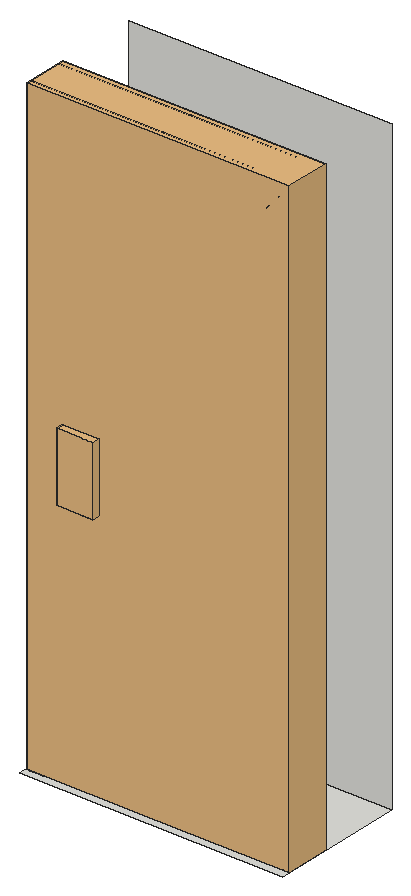
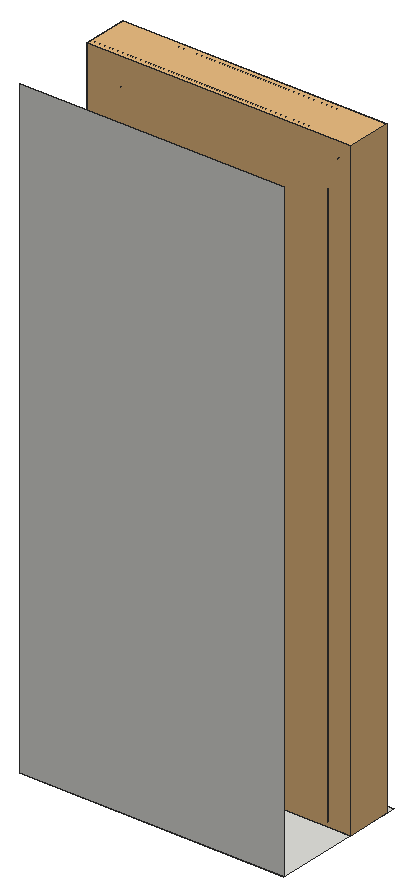
# SketchUp Ruby script. Lengths in inches.
U = 1.inch
M = Sketchup.active_model
def pt(a) = Geom::Point3d.new(a.map { |v| v * U })
def face(e, loops, mat)
  f = e.add_face(loops[0].map { |a| pt(a) })
  loops[1..].each { |l| e.add_face(l.map { |a| pt(a) }).erase! }
  f.material = f.back_material = mat if mat
  f
end
# faces: each face lists its corners as indices into pts; further lists are holes
def faces(e, pts, list, mat = nil) = list.each { |f| face(e, (f[0].is_a?(Array) ? f : [f]).map { |l| l.map { |i| pts[i] } }, mat) }
# xy, xz, yz: faces in a plane at the given z, y or x. An outline is a flat list of corners, or four numbers for a rectangle; further outlines are holes
def ring(l) = l.size == 4 ? [[l[0], l[1]], [l[2], l[1]], [l[2], l[3]], [l[0], l[3]]] : l.each_slice(2).to_a
def flat(e, list, mat, &to3) = list.each { |f| face(e, (f[0].is_a?(Array) ? f : [f]).map { |l| ring(l).map { |u, v| to3.(u, v) } }, mat) }
def xy(e, z, list, mat = nil) = flat(e, list, mat) { |x, y| [x, y, z] }
def xz(e, y, list, mat = nil) = flat(e, list, mat) { |x, z| [x, y, z] }
def yz(e, x, list, mat = nil) = flat(e, list, mat) { |y, z| [x, y, z] }
def lines(e, pts, list) = list.each { |a, b| e.add_line(pt(pts[a]), pt(pts[b])) }
# prism: a flat outline (further loops are holes) pulled along v
def prism(e, loops, v, mat = nil)
  f = face(e, loops, mat); d = Geom::Vector3d.new(v.map { |x| x * U })
  f.pushpull(f.normal.samedirection?(d) ? d.length : -d.length)
end
def box(e, o, s, mat = nil) = prism(e, [[o, [o[0] + s[0], o[1], o[2]], [o[0] + s[0], o[1] + s[1], o[2]], [o[0], o[1] + s[1], o[2]]]], [0, 0, s[2]], mat)
def at(x, y, z, deg = 0) = Geom::Transformation.translation(pt([x, y, z])) * Geom::Transformation.rotation(ORIGIN, Z_AXIS, deg.degrees)
def axes(o, x, y, z) = Geom::Transformation.new([*x, 0, *y, 0, *z, 0, *pt(o).to_a, 1])
def part(name) = M.definitions.add(name)
# library, detail: a bought-in or finely detailed component or shape, given as its bounding box
def library(name, o, s) = part(name).tap { |d| box(d.entities, o, s) }
def detail(e, o, s) = box(e.add_group.entities, o, s)
def put(e, d, t, mat = nil) = e.add_instance(d, t).tap { |i| i.material = mat if mat }
def group(e, t, mat = nil) = e.add_group.tap { |g| g.transformation = t; g.material = mat if mat }.entities
root = M.entities
M.materials.add("Material \#0").color = [86, 53, 35]
M.materials.add("Material \#1").color = [140, 140, 140]
c1 = library("3DGeom~3_Defintion",[-83.33,-500,-350],[620.1,1000,533.33])
c2 = part("3DGeom~18_Defintion")
xz(c2.entities,-241.71,[[-976.3,0,23.7,0,23.7,7.58],[-976.3,0,23.7,7.58,-976.3,7.58]],"Material \#0")
xz(c2.entities,241.71,[[-976.3,0,-976.3,7.58,23.7,7.58],[-976.3,0,23.7,7.58,23.7,0]],"Material \#0")
yz(c2.entities,23.7,[[-241.71,0,0,0,-241.71,7.58],[0,0,0,7.58,-241.71,7.58],[0,0,241.71,0,241.71,7.58],[0,0,241.71,7.58,0,7.58]],"Material \#0")
c3 = part("3DGeom~20_Defintion")
xy(c3.entities,0,[[-976.3,-241.71,-976.3,-223.46,23.7,-241.71],[23.7,-241.71,-976.3,-223.46,5.45,-223.46],[23.7,-241.71,5.45,-223.46,5.45,0],[23.7,-241.71,5.45,0,23.7,0],[-976.3,-223.46,-976.3,-211.85,5.45,-223.46],
  [5.45,-223.46,-976.3,-211.85,-6.16,-211.85],[5.45,-223.46,-6.16,-211.85,-6.16,0],[5.45,-223.46,-6.16,0,5.45,0],[-6.16,0,-6.16,211.85,5.45,223.46],[-6.16,0,5.45,223.46,5.45,0],
  [5.45,0,23.7,241.71,23.7,0],[5.45,0,5.45,223.46,23.7,241.71],[-976.3,211.85,-976.3,223.46,5.45,223.46],[-976.3,211.85,5.45,223.46,-6.16,211.85],[-976.3,223.46,-976.3,241.71,23.7,241.71],
  [-976.3,223.46,23.7,241.71,5.45,223.46]],"Material \#0")
c4 = part("3DGeom~22_Defintion")
xz(c4.entities,-210.625,[[-1016.13,2.47,-1016.13,9.96,-16.28,2.47],[-16.28,2.47,-1016.13,9.96,-16.28,9.96],[-1016.13,9.96,-1016.13,51.7,-16.28,51.7],[-1016.13,9.96,-16.28,51.7,-16.28,9.96],[-1016.13,51.7,-1016.13,72.71,-16.28,51.7]],"Material \#0")
xz(c4.entities,210.625,[[-1016.13,2.47,-16.28,2.47,-1016.13,9.96],[-16.28,2.47,-16.28,9.96,-1016.13,9.96],[-1016.13,9.96,-16.28,51.7,-1016.13,51.7],[-1016.13,9.96,-16.28,9.96,-16.28,51.7],[-1016.13,51.7,-16.28,51.7,-1016.13,72.71]],"Material \#0")
yz(c4.entities,-16.28,[[-210.625,2.47,-210.625,9.96,0,9.96],[-210.625,2.47,0,9.96,0,2.47],[0,2.47,0,9.96,210.625,2.47],[210.625,2.47,0,9.96,210.625,9.96],[-210.625,9.96,-210.625,51.7,0,51.7],
  [-210.625,9.96,0,51.7,0,9.96],[0,9.96,0,51.7,210.625,9.96],[210.625,9.96,0,51.7,210.625,51.7],[-210.625,51.7,0,72.71,0,51.7],[0,51.7,0,72.71,210.625,51.7]],"Material \#0")
p = [[-1016.13,-210.625,72.71],[-16.13,-210.77,73.09],[-16.28,-210.625,51.7],[-16.28,-210.625,51.7],[-16.13,-210.77,73.09],[-16.28,0,72.71],
  [-16.13,210.77,73.09],[-16.28,210.625,51.7],[-16.28,210.625,51.7],[-16.13,210.77,73.09],[-1016.13,210.625,72.71]]
faces(c4.entities,p,[[0,1,2],[3,4,5],[5,6,7],[8,9,10]],"Material \#0")
c5 = part("3DGeom~21_Defintion")
xy(c5.entities,73.08,[[-976.3,-241.71,23.7,-241.71,-976.3,-223.46],[23.7,-241.71,5.45,-223.46,-976.3,-223.46],[23.7,-241.71,23.7,0,5.45,-223.46],[5.45,-223.46,23.7,0,5.45,0],[23.7,0,23.7,241.71,5.45,223.46],
  [5.45,0,23.7,0,5.45,223.46],[-976.3,223.46,23.7,241.71,-976.3,241.71],[-976.3,223.46,5.45,223.46,23.7,241.71]],"Material \#0")
c6 = part("3DGeom~19_Defintion")
xy(c6.entities,0,[[-6.28,-215.79,-994.45,-208.55,-13.52,-208.55],[-994.45,-215.79,-994.45,-208.55,-6.28,-215.79],[-6.28,-215.79,-13.52,-208.55,-13.52,0],[-6.28,-215.79,-13.52,0,-6.28,0],[-13.52,0,-13.52,208.55,-6.28,215.79],
  [-13.52,0,-6.28,215.79,-6.28,0],[-994.45,208.55,-6.28,215.79,-13.52,208.55],[-994.45,208.55,-994.45,215.79,-6.28,215.79]],"Material \#0")
p = [[-13.52,-208.55,0],[-994.45,-208.55,0],[-994.45,-207.81,0.07],[-14.25,-207.81,0.07],[-13.52,-208.55,0],[-14.25,-207.81,0.07],
  [-14.25,0,0.07],[-13.52,0,0],[-13.52,208.55,0],[-14.25,207.81,0.07],[-13.52,208.55,0],[-14.25,207.81,0.07],
  [-994.45,207.81,0.07],[-994.45,208.55,0],[-994.45,-207.21,0.27],[-994.45,-207.21,0.27],[-14.86,-207.21,0.27],[-14.86,-207.21,0.27],
  [-14.86,0,0.27],[-14.86,0,0.27],[-14.86,0,0.27],[-14.86,0,0.27],[-14.86,207.21,0.27],[-14.86,207.21,0.27],
  [-994.45,207.21,0.27],[-994.45,207.21,0.27],[-14.86,-207.21,0.27],[-994.45,-207.21,0.27],[-994.45,-206.74,0.6],[-15.33,-206.74,0.6],
  [-14.86,-207.21,0.27],[-15.33,-206.74,0.6],[-15.33,0,0.6],[-14.86,0,0.27],[-14.86,207.21,0.27],[-15.33,206.74,0.6],
  [-14.86,207.21,0.27],[-15.33,206.74,0.6],[-994.45,206.74,0.6],[-994.45,207.21,0.27],[-994.45,-206.4,1.07],[-15.66,-206.4,1.07],
  [-15.66,-206.4,1.07],[-15.66,0,1.07],[-15.66,206.4,1.07],[-15.66,206.4,1.07],[-994.45,206.4,1.07],[-994.45,-206.2,1.68],
  [-15.86,-206.2,1.68],[-15.86,-206.2,1.68],[-15.86,0,1.68],[-15.86,206.2,1.68],[-15.86,206.2,1.68],[-994.45,206.2,1.68],
  [-994.45,-206.13,2.41],[-15.93,-206.13,2.41],[-15.93,-206.13,2.41],[-15.93,0,2.41],[-15.93,206.13,2.41],[-15.93,206.13,2.41],
  [-994.45,206.13,2.41],[-994.45,-206.13,71.16],[-994.45,-206.22,71.59],[-15.79,-206.28,71.53],[-15.79,-206.28,71.53],[-15.84,0,71.59],
  [-15.93,0,71.16],[-15.79,206.28,71.53],[-15.79,206.28,71.53],[-994.45,206.22,71.59],[-994.45,206.13,71.16],[-15.79,-206.28,71.53],
  [-994.45,-206.48,71.84],[-994.45,-206.9,71.93],[-15.16,-206.9,71.93],[-15.79,-206.28,71.53],[-15.79,-206.28,71.53],[-15.16,-206.9,71.93],
  [-15.16,0,71.93],[-994.45,-206.48,71.84],[-15.59,0,71.84],[-15.79,-206.28,71.53],[-15.59,0,71.84],[-15.79,206.28,71.53],
  [-15.16,206.9,71.93],[-15.59,0,71.84],[-15.79,206.28,71.53],[-994.45,206.48,71.84],[-15.79,206.28,71.53],[-15.16,206.9,71.93],
  [-994.45,206.9,71.93],[-994.45,206.48,71.84],[-15.79,206.28,71.53],[-994.45,-227.27,72.01],[5.41,-227.47,72.33],[4.78,-226.84,71.93],
  [4.78,-226.84,71.93],[5.41,-227.47,72.33],[5.21,0,72.01],[-994.45,-226.84,71.93],[-994.45,-227.27,72.01],[5.21,0,72.01],
  [4.78,0,71.93],[4.78,226.84,71.93],[5.21,0,72.01],[5.21,0,72.01],[5.41,227.47,72.33],[4.78,226.84,71.93],
  [5.41,227.47,72.33],[-994.45,227.27,72.01],[-994.45,227.27,72.01],[-994.45,226.84,71.93],[-994.45,-227.27,72.01],[-994.45,-227.53,72.27],
  [5.41,-227.47,72.33],[5.41,-227.47,72.33],[5.47,0,72.27],[5.21,0,72.01],[5.41,227.47,72.33],[5.41,227.47,72.33],
  [-994.45,227.53,72.27],[-994.45,227.27,72.01],[-994.45,-227.61,72.7],[-994.45,-227.61,74.4375],[-994.45,-227.61,74.4375],[5.55,-227.61,74.4375],
  [5.55,-227.61,74.4375],[5.55,0,74.4375],[5.55,0,72.7],[5.55,227.61,74.4375],[5.55,227.61,74.4375],[-994.45,227.61,74.4375],
  [-994.45,227.61,74.4375],[-994.45,227.61,72.7]]
faces(c6.entities,p,[[0,1,2],[2,3,0],[4,5,6],[6,7,4],[8,7,6],[6,9,8],[10,11,12],[12,13,10],
  [3,2,14],[15,16,3],[5,17,18],[19,6,5],[9,6,20],[21,22,9],[11,23,24],[25,12,11],
  [26,27,28],[28,29,26],[30,31,32],[32,33,30],[34,33,32],[32,35,34],[36,37,38],[38,39,36],
  [29,28,40],[40,41,29],[31,42,43],[43,32,31],[35,32,43],[43,44,35],[37,45,46],[46,38,37],
  [41,40,47],[47,48,41],[42,49,50],[50,43,42],[44,43,50],[50,51,44],[45,52,53],[53,46,45],
  [48,47,54],[54,55,48],[49,56,57],[57,50,49],[51,50,57],[57,58,51],[52,59,60],[60,53,52],
  [61,62,63],[64,65,66],[66,65,67],[68,69,70],[71,72,73],[73,74,75],[76,77,78],[62,79,63],
  [78,80,76],[81,82,65],[83,80,78],[78,84,83],[65,85,86],[68,87,69],[88,89,90],[90,91,92],
  [93,94,95],[96,97,98],[95,99,100],[101,102,96],[103,102,104],[105,106,103],[107,108,109],[110,111,107],
  [112,113,114],[115,116,117],[117,116,118],[119,120,121],[114,122,123],[124,125,114],[113,122,114],[115,126,127],
  [127,128,115],[115,128,116],[118,128,127],[127,129,118],[116,128,118],[119,130,131],[132,133,119],[119,133,120]],"Material \#0")
c7 = part("3DGeom~15_Defintion")
xy(c7.entities,0,[[-961.58,-251.9,-958.5,-248.8125,-961.58,-237.8],[-961.58,-251.9,28.8,-248.8125,-958.5,-248.8125],[-961.58,-251.9,36.25,-251.9,28.8,-248.8125],[36.25,-251.9,19.98,-239.99,28.8,-248.8125],[36.25,-251.9,22.16,-237.8,19.98,-239.99],
  [-958.5,-248.8125,-958.5,-237.8,-961.58,-237.8],[19.98,-239.99,22.16,-237.8,3.36,-223.37],[-958.5,-237.8,-958.5,-223.37,-961.58,-220.28],[-961.58,-237.8,-958.5,-237.8,-961.58,-220.28],[22.16,-237.8,4.64,-220.28,3.36,-223.37],
  [-958.5,-223.37,4.64,-220.28,-961.58,-220.28],[-958.5,-223.37,3.36,-223.37,4.64,-220.28],[5.29,-219.63,8.375,-218.35,5.29,0],[8.375,-218.35,8.375,0,5.29,0],[5.29,0,8.375,0,5.29,219.63],
  [8.375,0,8.375,218.35,5.29,219.63],[8.375,218.35,22.8125,237.15,5.29,219.63],[-961.58,220.28,-958.5,223.37,-961.58,237.8],[-961.58,220.28,3.36,223.37,-958.5,223.37],[-961.58,220.28,4.64,220.28,3.36,223.37],
  [4.64,220.28,19.98,239.99,3.36,223.37],[4.64,220.28,22.16,237.8,19.98,239.99],[-958.5,223.37,-958.5,237.8,-961.58,237.8],[-958.5,237.8,-958.5,248.8125,-961.58,251.9],[-961.58,237.8,-958.5,237.8,-961.58,251.9],
  [22.16,237.8,28.8,248.8125,19.98,239.99],[22.16,237.8,36.25,251.9,28.8,248.8125],[-958.5,248.8125,36.25,251.9,-961.58,251.9],[-958.5,248.8125,28.8,248.8125,36.25,251.9]],"Material \#0")
xy(c7.entities,7.48,[[-962.79,-238.36,23.37,-238.36,-962.79,-219.67],[23.37,-238.36,4.67,-219.67,-962.79,-219.67],[23.37,-238.36,23.37,0,4.67,-219.67],[4.67,-219.67,23.37,0,4.67,0],[23.37,0,23.37,238.36,4.67,219.67],
  [4.67,0,23.37,0,4.67,219.67],[-962.79,219.67,23.37,238.36,-962.79,238.36],[-962.79,219.67,4.67,219.67,23.37,238.36]],"Material \#0")
xy(c7.entities,63.5625,[[-962.79,-238.36,-962.79,-219.67,4.67,-219.67],[-962.79,-238.36,4.67,-219.67,23.37,-238.36],[23.37,-238.36,4.67,-219.67,23.37,0],[4.67,-219.67,4.67,0,23.37,0],[23.37,0,4.67,219.67,23.37,238.36],
  [4.67,0,4.67,219.67,23.37,0],[-962.79,219.67,-962.79,238.36,4.67,219.67],[4.67,219.67,-962.79,238.36,23.37,238.36]],"Material \#0")
xy(c7.entities,69.64,[[-962.79,-219.62,4.63,-219.62,-962.79,-200.32],[4.63,-219.62,-14.68,-200.32,-962.79,-200.32],[4.63,-219.62,4.63,0,-14.68,-200.32],[-14.68,-200.32,4.63,0,-14.68,0],[-14.68,0,4.63,0,-14.68,200.32],
  [4.63,0,4.63,219.62,-14.68,200.32],[-962.79,200.32,-14.68,200.32,4.63,219.62],[-962.79,200.32,4.63,219.62,-962.79,219.62]],"Material \#0")
xy(c7.entities,71.04,[[-961.58,-251.9,-958.5,-248.8125,28.8,-248.8125],[-961.58,-251.9,-961.58,-237.8,-958.5,-248.8125],[-961.58,-251.9,28.8,-248.8125,36.25,-251.9],[36.25,-251.9,19.98,-239.99,22.16,-237.8],[36.25,-251.9,28.8,-248.8125,19.98,-239.99],
  [-958.5,-248.8125,-961.58,-237.8,-958.5,-237.8],[19.98,-239.99,3.36,-223.37,22.16,-237.8],[-958.5,-237.8,-961.58,-220.28,-958.5,-223.37],[-961.58,-237.8,-961.58,-220.28,-958.5,-237.8],[22.16,-237.8,3.36,-223.37,4.64,-220.28],
  [-958.5,-223.37,-961.58,-220.28,4.64,-220.28],[-958.5,-223.37,4.64,-220.28,3.36,-223.37],[5.29,-219.63,5.29,0,8.375,-218.35],[8.375,-218.35,5.29,0,8.375,0],[5.29,0,5.29,219.63,8.375,0],
  [8.375,0,5.29,219.63,8.375,218.35],[8.375,218.35,5.29,219.63,22.8125,237.15],[-961.58,220.28,-958.5,223.37,3.36,223.37],[-961.58,220.28,-961.58,237.8,-958.5,223.37],[-961.58,220.28,3.36,223.37,4.64,220.28],
  [4.64,220.28,3.36,223.37,19.98,239.99],[4.64,220.28,19.98,239.99,22.16,237.8],[-958.5,223.37,-961.58,237.8,-958.5,237.8],[-958.5,237.8,-961.58,251.9,-958.5,248.8125],[-961.58,237.8,-961.58,251.9,-958.5,237.8],
  [22.16,237.8,19.98,239.99,28.8,248.8125],[22.16,237.8,28.8,248.8125,36.25,251.9],[-958.5,248.8125,-961.58,251.9,36.25,251.9],[-958.5,248.8125,36.25,251.9,28.8,248.8125]],"Material \#0")
xz(c7.entities,-238.36,[[-962.79,63.5625,23.37,63.5625,23.37,72.07],[-962.79,63.5625,23.37,72.07,-962.79,72.07]],"Material \#0")
xz(c7.entities,-219.67,[[-962.79,7.48,4.67,7.48,-962.79,63.5625],[4.67,7.48,4.67,63.5625,-962.79,63.5625]],"Material \#0")
xz(c7.entities,219.67,[[-962.79,7.48,-962.79,63.5625,4.67,7.48],[4.67,7.48,-962.79,63.5625,4.67,63.5625]],"Material \#0")
xz(c7.entities,238.36,[[-962.79,63.5625,-962.79,72.07,23.37,72.07],[-962.79,63.5625,23.37,72.07,23.37,63.5625]],"Material \#0")
yz(c7.entities,4.67,[[-219.67,7.48,0,7.48,-219.67,63.5625],[0,7.48,0,63.5625,-219.67,63.5625],[0,7.48,219.67,63.5625,0,63.5625],[0,7.48,219.67,7.48,219.67,63.5625]],"Material \#0")
yz(c7.entities,23.37,[[-238.36,63.5625,0,63.5625,-238.36,72.07],[0,63.5625,0,72.07,-238.36,72.07],[0,63.5625,238.36,63.5625,238.36,72.07],[0,63.5625,238.36,72.07,0,72.07]],"Material \#0")
p = [[36.9,-251.24,0],[37.21,0,-0.16],[34.125,0,-0.14],[36.9,251.24,0],[33.83,243.81,0.02],[33.83,-243.8,0.02],
  [22.8125,-237.15,0],[24.99,-234.97,-0.01],[5.375,-220.37,0],[23.37,-238.36,7.48],[4.67,-219.67,7.48],[4.67,-219.67,7.48],
  [23.37,-238.36,7.48],[23.37,-238.36,0],[4.67,-219.67,7.48],[23.37,-238.36,0],[5.375,-220.37,0],[5.375,-220.37,0],
  [23.37,-238.36,0],[5.29,-219.63,0],[8.375,-218.35,0],[-15.36,-199.64,1.62],[4.67,-219.67,7.48],[5.375,-220.37,0],
  [-13.8,-201.19,0.06],[5.375,-220.37,0],[5.375,-220.37,0],[-14.84,-200.15,0.58],[5.375,-220.37,0],[-13.8,-201.19,0.06],
  [-6.08,-208.92,0],[5.375,-220.37,0],[-13.8,-201.19,0.06],[-6.08,-208.92,0],[-13.8,-201.19,0.06],[5.375,-220.37,0],
  [-6.08,-208.92,0],[-13.8,-201.19,0.06],[-13.09,-201.91,0],[-6.08,-208.92,0],[-13.09,-201.91,0],[-13.8,-201.19,0.06],
  [-15.36,199.64,1.62],[4.67,219.67,7.48],[5.375,220.37,0],[-13.8,201.19,0.06],[5.375,220.37,0],[5.375,220.37,0],
  [4.67,219.67,7.48],[-14.84,200.15,0.58],[5.375,220.37,0],[-13.8,201.19,0.06],[-6.08,208.92,0],[-13.09,201.91,0],
  [-13.8,201.19,0.06],[-6.08,208.92,0],[-13.8,201.19,0.06],[5.375,220.37,0],[-6.08,208.92,0],[5.375,220.37,0],
  [-13.8,201.19,0.06],[-6.08,208.92,0],[-13.8,201.19,0.06],[-13.09,201.91,0],[8.375,218.35,0],[24.99,234.97,-0.01],
  [22.8125,237.15,0],[23.37,238.36,7.48],[23.37,238.36,0],[23.37,238.36,0],[5.375,220.37,0],[5.375,220.37,0],
  [23.37,238.36,7.48],[4.67,219.67,7.48],[5.375,220.37,0],[23.37,238.36,0],[23.37,238.36,7.48],[-13.8,-201.19,0.06],
  [-14.84,-200.15,0.58],[-14.38,-200.61,0.26],[-13.8,-201.19,0.06],[-13.8,-201.19,0.06],[-14.38,-200.61,0.26],[-13.8,201.19,0.06],
  [-14.84,200.15,0.58],[-13.8,201.19,0.06],[-14.38,200.61,0.26],[-14.38,200.61,0.26],[-13.8,201.19,0.06],[4.63,-219.62,69.64],
  [4.63,-219.62,69.64],[-15.42,-199.57,9.43],[-15.36,-199.64,1.62],[-15.16,-199.83,1.04],[-15.16,-199.83,1.04],[-15.16,199.83,1.04],
  [-15.36,199.64,1.62],[-15.16,199.83,1.04],[-15.42,199.57,9.43],[4.63,219.62,69.64],[4.67,219.67,7.48],[4.63,219.62,69.64],
  [4.63,-219.62,69.64],[4.67,-219.67,63.5625],[4.67,-219.67,63.5625],[4.67,-219.67,7.48],[-15.28,-199.71,69.25],[4.63,-219.62,69.64],
  [-15.42,-199.57,9.43],[-15.28,-199.71,69.25],[-15.42,-199.57,2.34],[-15.42,-199.57,2.34],[-15.42,199.57,2.34],[-15.42,199.57,9.43],
  [-15.28,199.71,69.25],[-15.28,199.71,69.25],[4.63,219.62,69.64],[4.63,219.62,69.64],[4.67,219.67,63.5625],[4.67,219.67,63.5625],
  [-15.42,199.57,2.34],[4.67,-219.67,63.5625],[4.63,-219.62,69.64],[4.67,219.67,7.48],[4.67,219.67,63.5625],[4.63,219.62,69.64],
  [4.63,-219.62,69.64],[-15.28,-199.71,69.25],[-15.28,-199.71,69.25],[-15.42,-199.57,48.99],[-15.42,-199.57,48.99],[-15.28,-199.71,69.25],
  [-15.42,199.57,48.99],[-15.28,199.71,69.25],[-15.28,199.71,69.25],[-15.42,199.57,48.99],[4.63,219.62,69.64],[4.63,-219.62,69.64],
  [23.37,-238.36,72.07],[4.67,-219.67,63.5625],[4.67,-219.67,63.5625],[23.37,-238.36,63.5625],[23.37,-238.36,72.07],[4.67,-219.67,63.5625],
  [5.24,-220.23,70.03],[23.37,-238.36,72.07],[23.37,-238.36,63.5625],[4.67,-219.67,63.5625],[4.67,-219.67,63.5625],[4.63,-219.62,69.64],
  [4.63,219.62,69.64],[23.37,238.36,72.07],[4.67,219.67,63.5625],[4.67,219.67,63.5625],[5.24,220.23,70.03],[4.63,219.62,69.64],
  [23.37,238.36,63.5625],[4.67,219.67,63.5625],[4.67,219.67,63.5625],[23.37,238.36,63.5625],[23.37,238.36,72.07],[4.67,219.67,63.5625],
  [23.37,238.36,72.07],[4.63,-219.62,69.64],[-14.68,-200.32,69.64],[-15.28,-199.71,69.25],[-15.28,-199.71,69.25],[-14.68,-200.32,69.64],
  [4.63,-219.62,69.64],[-15.28,199.71,69.25],[-14.68,200.32,69.64],[4.63,219.62,69.64],[4.63,219.62,69.64],[-14.68,200.32,69.64],
  [4.63,-219.62,69.64],[5.24,-220.23,70.03],[23.37,-238.36,72.07],[4.63,219.62,69.64],[5.24,220.23,70.03],[5.375,-220.37,72.07],
  [5.375,-220.37,72.07],[23.37,-238.36,72.07],[5.375,220.37,72.07],[23.37,238.36,72.07],[5.375,220.37,72.07],[33.83,-243.8,71.03],
  [36.9,-251.24,71.04],[22.8125,-237.15,71.04],[34.125,0,71.19],[37.21,0,71.2],[24.99,-234.97,71.05],[5.29,-219.63,71.04],
  [8.375,-218.35,71.04],[33.83,243.81,71.03],[36.9,251.24,71.04],[22.8125,237.15,71.04],[24.99,234.97,71.05],[8.375,218.35,71.04]]
faces(c7.entities,p,[[0,1,2],[1,3,4],[4,2,1],[2,5,0],[6,0,5],[5,7,6],[8,9,10],[11,12,13],
  [14,15,16],[17,18,9],[19,6,7],[7,20,19],[21,22,23],[24,21,25],[26,10,27],[28,27,29],
  [30,31,32],[33,34,35],[36,37,38],[39,40,41],[42,43,44],[45,42,46],[47,48,49],[50,49,51],
  [52,53,54],[55,56,57],[58,59,60],[61,62,63],[64,65,66],[43,67,68],[43,69,70],[71,72,73],
  [74,75,76],[3,66,65],[65,4,3],[77,78,21],[27,79,80],[81,82,78],[83,84,42],[85,86,84],
  [49,87,88],[10,89,27],[90,91,27],[92,93,27],[91,92,27],[78,94,21],[84,95,42],[96,97,49],
  [98,96,49],[99,98,49],[100,101,49],[21,102,103],[21,104,105],[21,106,107],[21,108,109],[91,110,92],
  [21,111,108],[42,112,113],[42,113,114],[42,115,116],[42,117,118],[42,119,43],[98,120,96],[10,121,122],
  [123,124,125],[126,127,91],[128,129,91],[108,130,131],[113,132,133],[134,135,98],[136,134,98],[137,138,139],
  [140,141,142],[143,142,144],[145,146,147],[148,144,149],[150,151,152],[153,154,155],[151,156,157],[158,159,160],
  [161,162,154],[163,164,165],[166,167,168],[169,170,171],[172,173,134],[174,175,176],[177,178,151],[142,179,144],
  [175,180,181],[178,182,151],[183,184,154],[185,186,187],[186,185,188],[188,189,186],[187,190,185],[190,187,191],
  [191,192,190],[189,188,193],[193,194,189],[195,196,197],[196,195,194],[194,193,196]],"Material \#0")
c8 = library("3DGeom~16_Defintion",[-962.62,-252.34,-11.22],[1000,504.68,93.46])
c9 = part("3DGeom~17_Defintion")
yz(c9.entities,-1908.8,[[-436.03,-21.87,-436.73,-21.5,-435.91,-21.83],[436.03,-21.87,435.91,-21.83,436.73,-21.5],[-435.91,-21.83,-436.73,-21.5,-436.15,-21.125],[-435.91,-21.83,-436.15,-21.125,-435.87,-21.72],[435.91,-21.83,435.87,-21.72,436.15,-21.125],
  [435.91,-21.83,436.15,-21.125,436.73,-21.5],[-436.73,-21.5,-484.73,-21.37,-436.15,-1.11],[-471.46,-21.5,-484.73,-21.37,-436.73,-21.5],[-477.2,-21.5,-484.73,-21.37,-471.46,-21.5],[-481.82,-21.5,-484.73,-21.37,-477.2,-21.5],
  [-436.73,-21.5,-436.15,-1.11,-436.15,-21.125],[436.73,-21.5,436.15,-21.125,471.46,-21.5],[471.46,-21.5,436.15,-21.125,477.2,-21.5],[477.2,-21.5,436.15,-21.125,499.98,-0.85],[477.2,-21.5,499.98,-0.85,481.82,-21.5],
  [481.82,-21.5,487.35,-21,484.73,-21.37],[481.82,-21.5,491.8,-19.52,487.35,-21],[481.82,-21.5,497.64,-13.67,491.8,-19.52],[481.82,-21.5,499.98,-0.85,497.64,-13.67],[-484.73,-21.37,-498.5,-11.58,-499.84,-0.37],
  [-484.73,-21.37,-499.84,-0.37,-499.4,-0.5],[-484.73,-21.37,-499.4,-0.5,-436.15,-1.11],[-484.73,-21.37,-493.63,-18.42,-498.5,-11.58],[-484.73,-21.37,-489.71,-20.375,-493.63,-18.42],[-484.73,-21.37,-487.35,-21,-489.71,-20.375],
  [436.15,-21.125,436.15,-1.11,436.73,-0.74],[436.15,-21.125,436.73,-0.74,499.98,-0.85],[487.35,-21,491.8,-19.52,489.71,-20.375],[-489.71,-20.375,-491.8,-19.52,-493.63,-18.42],[491.8,-19.52,495.21,-17.08,493.63,-18.42],
  [491.8,-19.52,497.64,-13.67,495.21,-17.08],[-493.63,-18.42,-496.54,-15.5,-498.5,-11.58],[-493.63,-18.42,-495.21,-17.08,-496.54,-15.5],[495.21,-17.08,497.64,-13.67,496.54,-15.5],[-496.54,-15.5,-497.64,-13.67,-498.5,-11.58],
  [497.64,-13.67,499.125,-9.22,498.5,-11.58],[497.64,-13.67,499.625,-3.69,499.125,-9.22],[497.64,-13.67,499.98,-0.85,499.625,-3.69],[-498.5,-11.58,-499.625,-3.69,-499.84,-0.37],[-498.5,-11.58,-499.5,-6.6,-499.625,-3.69],
  [-498.5,-11.58,-499.125,-9.22,-499.5,-6.6],[499.125,-9.22,499.625,-3.69,499.5,-6.6],[-499.625,-3.69,-499.98,-0.85,-500,-0.52],[-499.625,-3.69,-500,-0.52,-499.84,-0.37],[-436.15,-1.11,-499.4,-0.5,-471.46,-0.74],
  [-436.15,-1.11,-471.46,-0.74,-436.73,-0.74],[-436.15,-1.11,-436.73,-0.74,-435.91,-0.41],[-436.15,-1.11,-435.91,-0.41,-435.87,-0.52],[436.15,-1.11,435.87,-0.52,435.91,-0.41],[436.15,-1.11,435.91,-0.41,436.73,-0.74],
  [499.98,-0.85,436.73,-0.74,471.46,-0.74],[499.98,-0.85,471.46,-0.74,499.4,-0.5],[499.98,-0.85,499.4,-0.5,499.96,-0.41],[499.98,-0.85,499.96,-0.41,500,-0.52],[-436.73,-0.74,-436.03,-0.37,-435.91,-0.41],
  [436.73,-0.74,435.91,-0.41,436.03,-0.37],[-500,-0.52,-499.96,-0.41,-499.84,-0.37],[499.4,-0.5,499.84,-0.37,499.96,-0.41],[-499.84,141.21,-499.96,141.25,-499.4,141.35],[-436.03,141.21,-436.73,141.59,-435.91,141.25],
  [436.03,141.21,435.91,141.25,436.73,141.59],[499.84,141.21,484.73,162.21,498.5,152.42],[499.84,141.21,499.4,141.35,484.73,162.21],[499.84,141.21,498.5,152.42,499.625,144.53],[499.84,141.21,499.625,144.53,500,141.37],
  [499.84,141.21,500,141.37,499.96,141.25],[-499.96,141.25,-500,141.37,-499.98,141.69],[-499.96,141.25,-499.98,141.69,-499.4,141.35],[-435.91,141.25,-436.73,141.59,-436.15,141.96],[-435.91,141.25,-436.15,141.96,-435.87,141.37],
  [435.91,141.25,435.87,141.37,436.15,141.96],[435.91,141.25,436.15,141.96,436.73,141.59],[-499.4,141.35,-499.98,141.69,-471.46,141.59],[499.4,141.35,436.15,141.96,484.73,162.21],[499.4,141.35,471.46,141.59,436.15,141.96],
  [500,141.37,499.625,144.53,499.98,141.69],[-436.73,141.59,-499.98,141.69,-436.15,161.97],[-471.46,141.59,-499.98,141.69,-436.73,141.59],[-436.73,141.59,-436.15,161.97,-436.15,141.96],[436.73,141.59,436.15,141.96,471.46,141.59],
  [-499.98,141.69,-477.2,162.34,-436.15,161.97],[-499.98,141.69,-481.82,162.34,-477.2,162.34],[-499.98,141.69,-497.64,154.51,-481.82,162.34],[-499.98,141.69,-499.625,144.53,-497.64,154.51],[436.15,141.96,436.15,161.97,436.73,162.34],
  [436.15,141.96,436.73,162.34,484.73,162.21],[-499.625,144.53,-499.125,150.07,-497.64,154.51],[-499.625,144.53,-499.5,147.44,-499.125,150.07],[499.625,144.53,498.5,152.42,499.5,147.44],[499.5,147.44,498.5,152.42,499.125,150.07],
  [-499.125,150.07,-498.5,152.42,-497.64,154.51],[498.5,152.42,484.73,162.21,493.63,159.26],[498.5,152.42,493.63,159.26,496.54,156.34],[498.5,152.42,496.54,156.34,497.64,154.51],[-497.64,154.51,-491.8,160.36,-481.82,162.34],
  [-497.64,154.51,-495.21,157.92,-491.8,160.36],[-497.64,154.51,-496.54,156.34,-495.21,157.92],[496.54,156.34,493.63,159.26,495.21,157.92],[-495.21,157.92,-493.63,159.26,-491.8,160.36],[493.63,159.26,484.73,162.21,489.71,161.22],
  [493.63,159.26,489.71,161.22,491.8,160.36],[-491.8,160.36,-487.35,161.84,-481.82,162.34],[-491.8,160.36,-489.71,161.22,-487.35,161.84],[489.71,161.22,484.73,162.21,487.35,161.84],[-487.35,161.84,-484.73,162.21,-481.82,162.34],
  [-436.15,161.97,-477.2,162.34,-471.46,162.34],[-436.15,161.97,-471.46,162.34,-436.73,162.34],[-436.15,161.97,-436.73,162.34,-435.91,162.68],[-436.15,161.97,-435.91,162.68,-435.87,162.56],[436.15,161.97,435.87,162.56,435.91,162.68],
  [436.15,161.97,435.91,162.68,436.73,162.34],[484.73,162.21,436.73,162.34,471.46,162.34],[484.73,162.21,471.46,162.34,477.2,162.34],[484.73,162.21,477.2,162.34,481.82,162.34],[-436.73,162.34,-436.03,162.72,-435.91,162.68],
  [436.73,162.34,435.91,162.68,436.03,162.72]],"Material \#0")
xy(root,156.59,[[95.81,114.72,131.25,133.09]])
xz(root,115.85,[[101.96,191.32,101.96,191.45,101.97,191.44],[101.97,191.44,101.96,191.45,101.96,197.51],[101.97,191.44,101.96,197.51,101.96,199.18],[101.97,191.44,101.96,199.18,101.97,199.18]],"Material \#1")
xz(root,117.63,[[101.95,191.32,101.96,191.32,101.96,191.45],[101.96,191.32,101.97,191.44,101.96,191.45],[101.97,191.44,101.96,197.51,101.96,191.45],[101.97,191.44,101.96,199.18,101.96,197.51],[101.97,191.44,101.97,199.18,101.96,199.18]],"Material \#1")
xz(root,133.09,[[95.81,156.59,131.25,239.46]])
put(root,c1,axes([101.39,117.36,195.3125],[0.00787,0,0],[0,0,0.00929],[0,0.00737,0]),"Material \#1")
put(root,c2,axes([113.53,121.22,236.36],[0,0,0.08171],[0.06923,0,0],[0,-0.06476,0]),"Material \#0")
put(root,c3,axes([113.53,121.22,236.36],[0,0,0.08171],[0.06923,0,0],[0,-0.06476,0]),"Material \#0")
put(root,c4,axes([113.53,121.22,236.36],[0,0,0.07851],[0.06652,0,0],[0,-0.06222,0]),"Material \#0")
put(root,c5,axes([113.53,121.22,236.36],[0,0,0.08171],[0.06923,0,0],[0,-0.06476,0]),"Material \#0")
put(root,c6,axes([113.53,121.22,236.36],[0,0,0.08022],[0.06797,0,0],[0,-0.06357,0]),"Material \#0")
put(root,c7,axes([113.53,121.22,236.36],[0,0,0.08286],[0.07021,0,0],[0,-0.06566,0]),"Material \#0")
put(root,c8,axes([113.53,121.22,236.36],[0,0,0.08287],[0.07022,0,0],[0,-0.06568,0]),"Material \#0")
put(root,c9,axes([113.53,121.22,236.36],[0,0,0.04179],[0.03541,0,0],[0,-0.03312,0]),"Material \#0")
